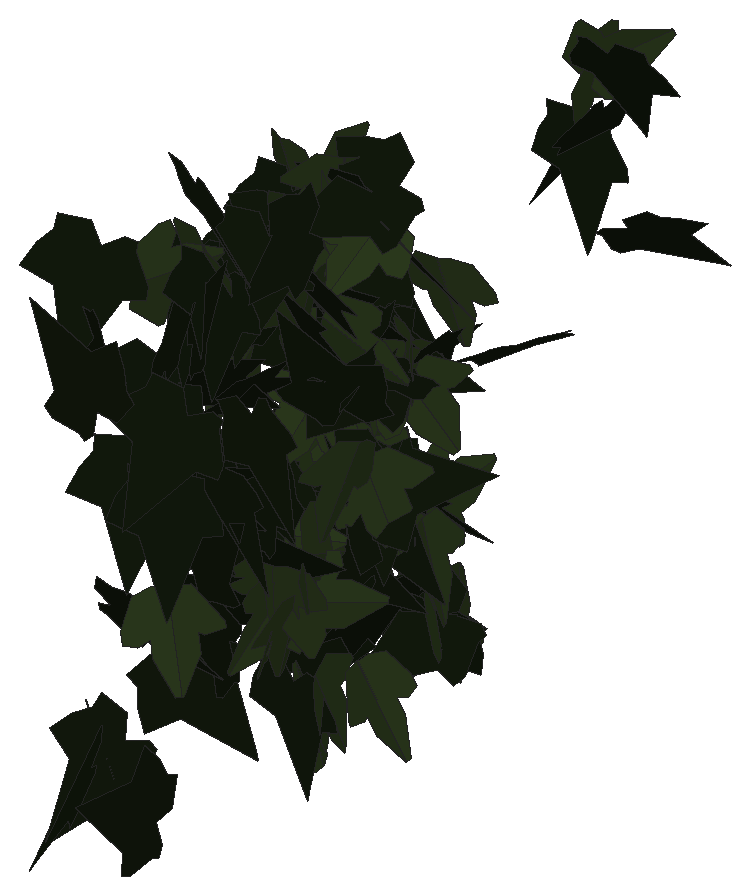
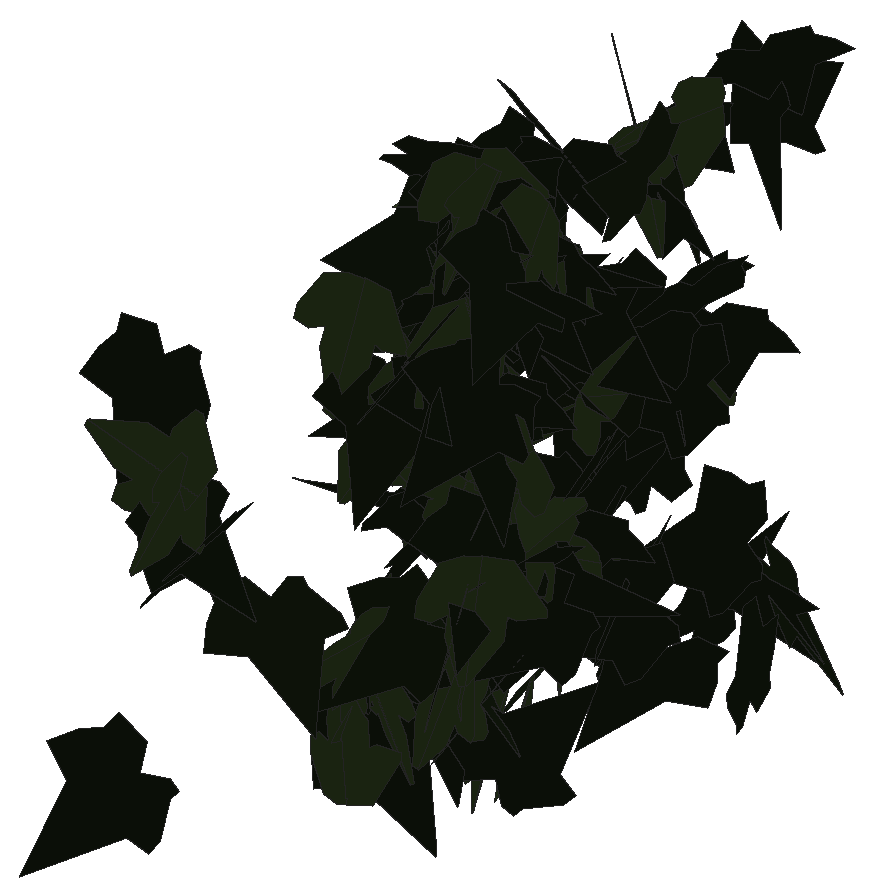
# SketchUp Ruby script. Lengths in inches.
U = 1.inch
M = Sketchup.active_model
def pt(a) = Geom::Point3d.new(a.map { |v| v * U })
def face(e, loops, mat)
  f = e.add_face(loops[0].map { |a| pt(a) })
  loops[1..].each { |l| e.add_face(l.map { |a| pt(a) }).erase! }
  f.material = f.back_material = mat if mat
  f
end
# faces: each face lists its corners as indices into pts; further lists are holes
def faces(e, pts, list, mat = nil) = list.each { |f| face(e, (f[0].is_a?(Array) ? f : [f]).map { |l| l.map { |i| pts[i] } }, mat) }
# xy, xz, yz: faces in a plane at the given z, y or x. An outline is a flat list of corners, or four numbers for a rectangle; further outlines are holes
def ring(l) = l.size == 4 ? [[l[0], l[1]], [l[2], l[1]], [l[2], l[3]], [l[0], l[3]]] : l.each_slice(2).to_a
def flat(e, list, mat, &to3) = list.each { |f| face(e, (f[0].is_a?(Array) ? f : [f]).map { |l| ring(l).map { |u, v| to3.(u, v) } }, mat) }
def xy(e, z, list, mat = nil) = flat(e, list, mat) { |x, y| [x, y, z] }
def xz(e, y, list, mat = nil) = flat(e, list, mat) { |x, z| [x, y, z] }
def yz(e, x, list, mat = nil) = flat(e, list, mat) { |y, z| [x, y, z] }
def lines(e, pts, list) = list.each { |a, b| e.add_line(pt(pts[a]), pt(pts[b])) }
# prism: a flat outline (further loops are holes) pulled along v
def prism(e, loops, v, mat = nil)
  f = face(e, loops, mat); d = Geom::Vector3d.new(v.map { |x| x * U })
  f.pushpull(f.normal.samedirection?(d) ? d.length : -d.length)
end
def box(e, o, s, mat = nil) = prism(e, [[o, [o[0] + s[0], o[1], o[2]], [o[0] + s[0], o[1] + s[1], o[2]], [o[0], o[1] + s[1], o[2]]]], [0, 0, s[2]], mat)
def at(x, y, z, deg = 0) = Geom::Transformation.translation(pt([x, y, z])) * Geom::Transformation.rotation(ORIGIN, Z_AXIS, deg.degrees)
def axes(o, x, y, z) = Geom::Transformation.new([*x, 0, *y, 0, *z, 0, *pt(o).to_a, 1])
def part(name) = M.definitions.add(name)
# library, detail: a bought-in or finely detailed component or shape, given as its bounding box
def library(name, o, s) = part(name).tap { |d| box(d.entities, o, s) }
def detail(e, o, s) = box(e.add_group.entities, o, s)
def put(e, d, t, mat = nil) = e.add_instance(d, t).tap { |i| i.material = mat if mat }
def group(e, t, mat = nil) = e.add_group.tap { |g| g.transformation = t; g.material = mat if mat }.entities
root = M.entities
M.materials.add("efeu1").color = [18, 25, 13]
M.materials.add("efeu2").color = [43, 57, 29]
c1 = part("ivyleaf_9")
p = [[1.54,2.16,1.25],[1.36,2.04,1.19],[-0.21,0.99,0.68],[-0.71,1.11,0.82],[-0.85,0.86,0.67],[-0.8,0.17,0.21],
  [-0.9,-0.01,0.1],[-0.67,-0.16,-0.02],[-0.08,-0.08,-0.05],[-0.03,-0.6,-0.4],[0.65,-0.88,-0.66],[0.83,-0.6,-0.49],
  [1.29,-0.42,-0.43],[1.8125,-0.07,-0.26],[1.21,0.44,0.15]]
faces(c1.entities,p,[[0,1,2,3,4,5,6,7,8,9,10,11,12,13,14]],"efeu1")
c2 = part("ivyleaf_10")
p = [[0,0.5,-0.03],[-0.0625,2.02,-0.43],[-0.19,2.01,-0.46],[-0.54,1.05,-0.29],[-0.52,0.625,-0.18],[-0.83,0.76,-0.28],
  [-1.16,0.64,-0.33],[-1.15,0.33,-0.24],[-0.77,-0.39,0.02],[-0.3,-0.51,0.16],[0.04,-0.48,0.23],[-0.02,2.01,-0.4375],
  [-0.06,2.01,-0.43],[0.04,-0.49,0.23],[0.67,-0.49,0.14],[1.38,0.36,-0.2],[1.375,0.51,-0.24],[0.81,0.65,-0.19],
  [0.62,0.59,-0.15],[0.6,1.09,-0.28],[0.5,1.23,-0.31]]
faces(c2.entities,p,[[0,1,2,3,4,5,6,7,8,9,10],[11,12,0,13,14,15,16,17,18,19,20]],"efeu2")
put(root,c1,axes([51.26,220.86,248.3],[0.28668,-0.3638,0.18833],[0.11725,-0.14738,-0.46318],[0.39252,0.30973,0.00081]))
put(root,c2,axes([51.57,222.2,244.75],[-0.11598,0.036,-0.48503],[-0.02936,-0.49824,-0.02996],[-0.48548,0.02153,0.11769]))
put(root,c1,axes([51.99,221.61,243.91],[-0.31629,0.04961,0.38406],[-0.38199,0.04146,-0.31994],[-0.06359,-0.4958,0.01167]))
put(root,c1,axes([51.36,223.23,243.51],[0.19328,-0.46108,0.00663],[0.00595,-0.0047,-0.49994],[0.46109,0.19334,0.00367]))
put(root,c2,axes([51.57,222.15,248.25],[-0.43953,0.21947,-0.09299],[0.07231,-0.0631,-0.4907],[-0.22712,-0.44481,0.02373]))
put(root,c2,axes([51.52,221.34,245.96],[-0.0779,-0.19546,0.45357],[0.19442,-0.43424,-0.15374],[0.45402,0.15241,0.14365]))
put(root,c1,axes([51.76,221.43,246.8],[-0.06436,0.17689,-0.46322],[0.04543,-0.46303,-0.18313],[-0.49375,-0.06566,0.04353]))
put(root,c1,axes([51.73,222.36,247.43],[-0.42644,-0.26019,-0.02116],[0.01619,0.01409,-0.49954],[0.26054,-0.42674,-0.00359]))
put(root,c1,axes([51.6,218.64,248.58],[-0.25307,-0.42792,-0.05328],[0.03038,0.04393,-0.49714],[0.43015,-0.25486,0.00377]))
put(root,c1,axes([51.46,219.9,246.58],[0.0908,-0.44479,-0.20957],[0.01331,0.21525,-0.4511],[0.49151,0.07635,0.05093]))
put(root,c2,axes([51.7,222.9,244.55],[-0.37664,-0.32541,-0.04743],[0.03783,0.02876,-0.49774],[0.32666,-0.37853,0.00296]))
put(root,c1,axes([51.77,222.17,247.75],[0.14094,0.44731,0.17335],[-0.02008,0.18602,-0.46368],[-0.4793,0.12374,0.0704]))
put(root,c1,axes([51.48,218.97,241.69],[-0.0454,-0.08304,0.49096],[0.13869,-0.4756,-0.06761],[0.47823,0.13005,0.06621]))
put(root,c1,axes([51.89,221.84,247.4375],[-0.40379,-0.19244,0.22343],[-0.14678,-0.19742,-0.43529],[0.25575,-0.41712,0.10294]))
put(root,c1,axes([51.32,219.3125,243.56],[0.42437,-0.11959,0.23581],[0.22597,-0.0675,-0.44089],[0.13728,0.48077,-0.00324]))
put(root,c1,axes([51.73,221.92,247.89],[-0.42595,-0.14972,-0.21483],[0.20764,0.05681,-0.45129],[0.15954,-0.47366,0.01378]))
put(root,c2,axes([52.01,220.06,247.96],[-0.39785,0.09308,0.28819],[-0.28916,0.02467,-0.40716],[-0.09001,-0.49064,0.0342]))
put(root,c1,axes([51.56,221.83,243.89],[0.41357,0.21089,0.1857],[0.15818,0.09838,-0.464],[-0.23224,0.44255,0.01466]))
put(root,c1,axes([51.67,220.26,247.77],[-0.33369,-0.1402,-0.34496],[0.34602,0.05436,-0.35681],[0.13755,-0.47685,0.06075]))
put(root,c1,axes([52.04,222.14,242],[0.16265,-0.00759,0.47275],[-0.46684,0.07659,0.16185],[-0.07488,-0.49404,0.01783]))
put(root,c1,axes([51.74,222.03,247.49],[-0.15012,0.09118,-0.46814],[0.34568,-0.31732,-0.17266],[-0.32859,-0.37549,0.03223]))
put(root,c1,axes([51.67,222.49,244.45],[-0.07447,-0.49405,0.01914],[0.05289,-0.0272,-0.49645],[0.49159,-0.07192,0.05632]))
put(root,c1,axes([51.63,220.11,242.6],[-0.01615,-0.25594,-0.42922],[0.07399,0.42349,-0.25531],[0.49423,-0.07177,0.0242]))
put(root,c1,axes([51.91,222.375,244.79],[0.15371,0.47271,0.05406],[-0.00337,0.05789,-0.49663],[-0.47577,0.15231,0.02098]))
put(root,c2,axes([51.51,222.42,245.81],[0.28931,-0.03294,0.40647],[0.40683,0.05764,-0.28489],[-0.02809,0.49557,0.06015]))
put(root,c1,axes([51.74,221.39,244.57],[-0.28529,-0.31507,-0.26332],[0.21986,0.1536,-0.42198],[0.3468,-0.35656,0.0509]))
put(root,c1,axes([51.75,220.09,246.3],[0.3452,0.3229,0.16302],[0.10935,0.12164,-0.47249],[-0.34479,0.36186,0.01336]))
put(root,c1,axes([51.5625,220.45,243.26],[0.40562,0.07389,0.28286],[0.27079,0.0874,-0.41114],[-0.1102,0.48672,0.03088]))
put(root,c1,axes([52.06,222.32,246.23],[-0.06487,0.49409,-0.04086],[0.01115,-0.03974,-0.49829],[-0.49565,-0.06556,-0.00586]))
put(root,c1,axes([51.73,228.15,244.72],[0.42356,0.23625,0.1216],[0.07732,0.10933,-0.48173],[-0.25421,0.42689,0.05608]))
put(root,c1,axes([52.05,217.88,242.33],[-0.38188,0.24669,-0.20811],[0.178,-0.10796,-0.4546],[-0.26923,-0.42129,-0.00536]))
put(root,c1,axes([51.95,220.89,244.33],[-0.10654,-0.15839,0.46213],[-0.20153,-0.41662,-0.18925],[0.44501,-0.22659,0.02493]))
put(root,c1,axes([51.78,220.84,245.13],[0.29553,-0.29838,-0.27135],[-0.16163,0.22059,-0.41859],[0.36951,0.33513,0.03393]))
put(root,c1,axes([52.15,218.03,247.79],[0.18574,0.03141,-0.46316],[-0.46216,-0.0344,-0.18768],[-0.04365,0.49783,0.01626]))
put(root,c1,axes([52.09,218.4375,242.45],[-0.47247,-0.16016,-0.03354],[0.03292,0.00734,-0.49886],[0.16029,-0.4736,0.00361]))
put(root,c2,axes([51.95,227.12,247.35],[-0.01205,-0.26423,-0.42431],[0.07235,0.41904,-0.26301],[0.49459,-0.06773,0.02813]))
put(root,c1,axes([52.04,222.67,244.3],[0.23102,-0.05226,-0.44034],[-0.39507,0.20122,-0.23115],[0.20137,0.45473,0.05168]))
put(root,c1,axes([51.89,219.03,245.73],[-0.31854,-0.31751,-0.21845],[0.16814,0.14052,-0.44942],[0.34679,-0.35978,0.01725]))
put(root,c1,axes([51.86,222.4375,246.45],[0.34188,0.34864,0.10756],[0.0691,0.08286,-0.48822],[-0.35825,0.34869,0.00847]))
put(root,c1,axes([51.91,220.52,245.91],[0.25705,0.31685,0.28902],[0.09313,0.28768,-0.3982],[-0.41863,0.25855,0.08888]))
put(root,c2,axes([51.83,219.25,248.07],[0.02127,-0.04023,-0.49792],[0.24173,0.43697,-0.02498],[0.43717,-0.23966,0.03804]))
put(root,c1,axes([52.11,219.22,247.04],[0.10233,0.07979,0.48287],[-0.06366,0.49129,-0.06769],[-0.48526,-0.04763,0.11071]))
put(root,c1,axes([51.96,220.5625,242.76],[-0.09802,0.00982,0.4902],[-0.12214,-0.48463,-0.01472],[0.47484,-0.12263,0.09741]))
put(root,c2,axes([52.0625,222.24,244.76],[-0.24033,-0.43536,0.05199],[0.01082,-0.06515,-0.49562],[0.43832,-0.2371,0.04074]))
put(root,c1,axes([51.76,219.38,245.18],[0.2831,0.11945,0.39445],[0.3145,0.24666,-0.30041],[-0.26636,0.4182,0.06452]))
put(root,c2,axes([51.96,221.76,247.84],[-0.47137,0.07466,-0.14912],[0.14341,-0.04673,-0.47671],[-0.08512,-0.49218,0.02264]))
put(root,c2,axes([51.97,221.51,247.5],[-0.46904,-0.04817,-0.16638],[0.17246,-0.08512,-0.46153],[0.01614,-0.49034,0.09646]))
put(root,c1,axes([51.99,222.3,246.36],[-0.32942,-0.28337,-0.24736],[0.19344,0.15436,-0.43446],[0.32259,-0.38194,0.00793]))
put(root,c1,axes([52.375,217.59,247.29],[0.0705,0.01386,0.49481],[-0.38445,0.31636,0.04592],[-0.31181,-0.38694,0.05526]))
put(root,c1,axes([52.25,226.92,246.97],[-0.21855,0.32414,-0.31172],[0.09747,-0.3042,-0.38466],[-0.43902,-0.2289,0.06978]))
put(root,c1,axes([51.84,221.69,247.38],[0.41578,-0.27673,-0.02335],[-0.02395,0.00614,-0.49939],[0.27668,0.41639,-0.00815]))
put(root,c2,axes([51.91,222.75,243.16],[0.00176,0.00965,0.4999],[0.31323,-0.38967,0.00642],[0.38972,0.31315,-0.00741]))
put(root,c2,axes([52.13,222.82,243.3],[-0.46407,0.17339,-0.06761],[0.06695,-0.01394,-0.4953],[-0.17365,-0.46877,-0.01028]))
put(root,c1,axes([51.97,226.96,246.55],[0.04959,-0.48818,0.09603],[0.03004,-0.09339,-0.49028],[0.49663,0.05439,0.02007]))
put(root,c1,axes([52.55,221.65,246.53],[-0.42631,0.13349,0.2246],[-0.20918,0.08314,-0.44646],[-0.15654,-0.47463,-0.01504]))
put(root,c2,axes([52.23,222.15,248.34],[-0.10709,0.38107,0.30548],[-0.1097,0.28598,-0.3952],[-0.47592,-0.15167,0.02236]))
put(root,c2,axes([52.21,222.38,247.12],[0.2655,0.40604,-0.12101],[-0.11442,-0.06879,-0.48185],[-0.40794,0.28355,0.05639]))
put(root,c2,axes([52.23,222.05,247.87],[0.27671,0.37306,-0.18507],[-0.11622,-0.1442,-0.46444],[-0.3999,0.30005,0.00691]))
put(root,c2,axes([52.19,221.78,245.47],[-0.31276,-0.18893,0.34131],[0.16621,-0.46029,-0.10249],[0.35293,0.04934,0.35072]))
put(root,c2,axes([51.91,221.17,243.97],[0.04759,-0.14933,-0.4748],[0.49585,0.05567,0.03219],[0.04325,-0.47392,0.15339]))
put(root,c2,axes([52.0625,227.1,247.41],[-0.21353,-0.21142,0.39963],[0.29474,0.27003,0.30034],[-0.34283,0.36385,0.00931]))
put(root,c1,axes([52.59,224.96,244.93],[-0.00337,0.48882,-0.10508],[-0.20225,-0.09743,-0.44677],[-0.45726,0.0395,0.19838]))
put(root,c2,axes([52.43,222.03,248.41],[-0.3809,-0.31944,0.05355],[-0.03692,-0.03931,-0.49708],[0.32179,-0.38264,0.00636]))
put(root,c1,axes([52.08,222.33,245],[0.11628,-0.37991,0.30356],[0.09467,-0.28846,-0.39728],[0.47699,0.14987,0.00485]))
put(root,c1,axes([52.29,221.95,248.28],[0.44401,0.17074,-0.15397],[-0.14537,-0.05093,-0.47568],[-0.17812,0.46718,0.00441]))
put(root,c1,axes([52.11,219.74,244.18],[-0.12351,0.01114,0.48438],[0.33492,-0.35924,0.09366],[0.35011,0.34759,0.08128]))
put(root,c2,axes([52.48,220.72,243.25],[0.19398,-0.38193,-0.25787],[-0.08536,0.24517,-0.42732],[0.45287,0.20981,0.02991]))
put(root,c1,axes([52.4,220.68,248.08],[-0.36743,-0.29294,-0.17083],[0.14231,0.09544,-0.46972],[0.30781,-0.3938,0.01324]))
put(root,c1,axes([52.76,220.35,244.73],[-0.04003,0.03925,0.49685],[-0.32741,0.37373,-0.0559],[-0.37576,-0.32983,-0.00421]))
put(root,c2,axes([52.5,221.27,247.24],[0.01912,-0.49947,0.01288],[-0.00464,-0.01306,-0.49981],[0.49961,0.019,-0.00513]))
put(root,c1,axes([52.31,219.49,247.3],[-0.10787,0.30262,0.38313],[0.08094,-0.37585,0.31966],[0.48147,0.13098,0.03209]))
put(root,c1,axes([52.29,219.93,247.83],[0.01876,-0.48647,0.11398],[0.01419,-0.11349,-0.48674],[0.49945,0.0215,0.00955]))
put(root,c1,axes([52.78,222.08,243.34],[-0.35042,0.35405,0.04309],[-0.03887,0.02213,-0.498],[-0.35454,-0.35236,0.01202]))
put(root,c2,axes([52.53,220.73,243.45],[0.0766,0.29903,-0.39334],[-0.12312,-0.37393,-0.30825],[-0.47851,0.14408,0.01634]))
put(root,c2,axes([52.64,220.54,243.84],[-0.46703,-0.17385,0.04069],[-0.03597,-0.01999,-0.4983],[0.17489,-0.46838,0.00617]))
put(root,c2,axes([52.35,222.29,245.03],[0.44714,0.1249,0.18566],[0.17503,0.06322,-0.46408],[-0.1394,0.48,0.01281]))
put(root,c1,axes([52.52,222.36,247.24],[-0.21886,-0.44921,0.01771],[0.01017,-0.02464,-0.49929],[0.44944,-0.21818,0.01992]))
put(root,c1,axes([52.34,220.93,247.23],[0.49735,-0.04345,-0.02755],[-0.02725,0.00463,-0.49924],[0.04364,0.49809,0.00224]))
put(root,c1,axes([52.35,222.96,243.875],[0.49185,0.06989,0.05654],[0.0422,0.09822,-0.48844],[-0.07938,0.48525,0.09072]))
put(root,c1,axes([52.43,222.4,247.02],[0.30693,-0.2732,-0.28488],[-0.12078,0.27856,-0.39726],[0.37577,0.31268,0.105]))
put(root,c2,axes([52.71,221.14,241.46],[-0.2052,0.45084,-0.06805],[-0.03799,0.05746,0.49523],[0.45437,0.20842,0.01067]))
put(root,c1,axes([52.28,221.73,243.62],[0.02211,0.0454,-0.49744],[0.30806,0.39072,0.04936],[0.39321,-0.30866,-0.01069]))
put(root,c1,axes([52.68,218.27,241.73],[-0.04028,-0.02414,0.49779],[-0.2589,-0.42573,-0.04159],[0.42585,-0.2611,0.02179]))
put(root,c2,axes([52.76,223.12,243.18],[0.38683,-0.22506,-0.22295],[-0.17791,0.13682,-0.4468],[0.26212,0.425,0.02577]))
put(root,c1,axes([52.41,219.875,245.39],[0.25741,-0.42864,0.00309],[0.00043,-0.00334,-0.49999],[0.42865,0.25741,-0.00135]))
put(root,c1,axes([52.42,221.47,246.99],[0.45884,0.14378,0.13709],[0.12035,0.07331,-0.47973],[-0.15805,0.47324,0.03267]))
put(root,c2,axes([52.71,220.77,243.42],[0.05781,-0.49662,0.00469],[0.00271,-0.00441,-0.49997],[0.49664,0.05783,0.00218]))
put(root,c1,axes([52.55,218.77,245.7],[-0.06614,-0.49369,-0.04356],[0.00564,0.04319,-0.4981],[0.49557,-0.06638,-0.00015]))
put(root,c2,axes([52.74,221.31,242.1],[-0.16167,0.42183,0.2143],[-0.12658,0.17965,-0.44911],[-0.45589,-0.19947,0.04871]))
put(root,c1,axes([52.29,220.64,244.05],[0.14779,-0.18467,0.44051],[0.40939,-0.18858,-0.21641],[0.24608,0.42465,0.09546]))
put(root,c1,axes([52.87,222.07,242.98],[-0.02076,0.48289,-0.128],[0.01699,-0.12735,-0.48321],[-0.49928,-0.02441,-0.01112]))
put(root,c1,axes([52.99,220.63,248.4],[-0.47735,0.14058,-0.0487],[0.04526,-0.01867,-0.4976],[-0.14173,-0.47947,0.0051]))
put(root,c1,axes([53.01,222.11,246.08],[-0.48579,-0.092,0.07447],[-0.07533,-0.00232,-0.49429],[0.0913,-0.49146,-0.0116]))
put(root,c2,axes([52.76,223.32,243.72],[0.14182,0.01797,-0.47913],[0.11275,0.48439,0.05153],[0.46602,-0.12266,0.13334]))
put(root,c1,axes([52.52,222.25,246.03],[0.16938,-0.03691,-0.46899],[0.14957,0.47682,0.01649],[0.44603,-0.14588,0.17257]))
put(root,c1,axes([52.6,220.93,242.29],[0.09851,-0.47136,0.1346],[0.05386,-0.12605,-0.48084],[0.48723,0.10924,0.02594]))
put(root,c1,axes([53.11,222.09,248.42],[-0.45182,-0.07812,0.1994],[-0.17779,-0.12269,-0.45093],[0.11938,-0.47838,0.08308]))
put(root,c1,axes([52.61,220.17,246.07],[0.22118,-0.44713,-0.03396],[-0.01142,0.03224,-0.49883],[0.44827,0.22143,0.00405]))
put(root,c2,axes([52.87,220.84,244.14],[0.1199,-0.19959,-0.44248],[0.0082,0.45655,-0.20371],[0.48534,0.04159,0.11276]))
put(root,c1,axes([52.83,226.36,248.14],[0.41987,0.18503,-0.19867],[-0.17541,-0.09437,-0.45861],[-0.20721,0.45482,-0.01433]))
put(root,c1,axes([53.1,222.79,242.5],[0.15279,0.23609,-0.41342],[-0.239,-0.33747,-0.28105],[-0.41174,0.2835,0.00973]))
put(root,c2,axes([52.96,221.95,247.8125],[-0.49788,-0.03148,0.03351],[0.02699,-0.49513,-0.06418],[0.03722,-0.06209,0.49473]))
put(root,c1,axes([52.84,220.69,247.86],[0.47118,0.05305,-0.15867],[-0.16197,0.02591,-0.47233],[-0.04189,0.4965,0.0416]))
put(root,c2,axes([53.02,222.34,246.07],[-0.16766,-0.44774,0.14634],[-0.00556,-0.15344,-0.47584],[0.47102,-0.16119,0.04647]))
put(root,c1,axes([53.08,222.5,245.96],[0.10217,0.47271,0.12689],[-0.00057,0.12974,-0.48287],[-0.48945,0.09853,0.02705]))
put(root,c2,axes([52.93,223.36,242.1875],[-0.47662,0.03841,0.14614],[0.14569,-0.01145,0.47817],[0.04008,0.49839,-0.00027]))
put(root,c2,axes([52.81,220.88,243.49],[0.00747,-0.15363,-0.47576],[0.32042,0.36671,-0.11338],[0.38376,-0.30319,0.10393]))
put(root,c1,axes([52.88,222.1875,244.8],[-0.11824,-0.47268,-0.11223],[0.05889,0.10071,-0.4862],[0.48224,-0.12819,0.03185]))
put(root,c2,axes([52.87,218.29,244.54],[0.44439,0.18474,0.13561],[0.12959,0.04144,-0.48113],[-0.18901,0.46277,-0.01106]))
put(root,c1,axes([53.1,218.3,247.07],[-0.27791,-0.41013,0.06749],[-0.04133,-0.05352,-0.49541],[0.41359,-0.28094,-0.00416]))
put(root,c1,axes([53.36,222.83,242.6],[-0.46791,-0.12654,0.12266],[-0.11194,-0.05539,-0.48415],[0.13612,-0.48054,0.02351]))
put(root,c1,axes([53.41,221.29,246.76],[-0.37151,0.3346,-0.00504],[0.00383,-0.00329,-0.49997],[-0.33461,-0.37153,-0.00012]))
put(root,c1,axes([53.3,220.89,246.19],[0.28975,-0.05918,0.40316],[-0.39268,0.09157,0.29566],[-0.10883,-0.48797,0.00659]))
put(root,c1,axes([52.98,221.9,244.35],[0.25363,-0.33578,-0.27005],[-0.09163,0.26416,-0.41452],[0.42104,0.25975,0.07247]))
put(root,c2,axes([53.16,222.23,246.28],[0.3803,-0.316,-0.0743],[0.03021,0.1484,-0.47651],[0.32321,0.35794,0.13197]))
put(root,c2,axes([53.1875,222.77,242.71],[-0.18885,0.45321,0.09453],[-0.02617,0.09148,-0.49086],[-0.46223,-0.19034,-0.01083]))
put(root,c1,axes([52.83,222.34,247.61],[0.37154,-0.26215,0.20793],[0.18771,-0.09393,-0.45381],[0.27699,0.41528,0.02862]))
put(root,c2,axes([53.04,222.45,245.67],[0.26877,0.31206,0.28352],[0.1275,0.26033,-0.4074],[-0.40188,0.29129,0.06037]))
put(root,c2,axes([53.11,221.66,244.83],[0.24673,0.39913,0.17269],[0.04058,0.17655,-0.46603],[-0.43298,0.24399,0.05473]))
put(root,c2,axes([53.26,221.1,245.37],[-0.03499,-0.46761,0.17355],[0.03103,-0.17568,-0.46709],[0.49781,-0.02192,0.04132]))
put(root,c2,axes([53.19,222.64,243.63],[-0.1163,0.48611,-0.01295],[0.00341,-0.0125,-0.49983],[-0.48627,-0.11635,-0.00041]))
put(root,c1,axes([52.88,221.99,244.52],[0.43278,-0.14843,-0.20166],[0.16183,0.47309,-0.0009],[0.19108,-0.06449,0.45753]))
put(root,c2,axes([53.28,222.81,247.05],[-0.49664,-0.04057,-0.0413],[0.04125,0.00236,-0.49829],[0.04063,-0.49835,0.001]))
put(root,c1,axes([53.35,221.96,246.17],[-0.4558,-0.14216,0.14845],[0.08629,-0.46011,-0.17565],[0.18655,-0.1345,0.44397]))
put(root,c2,axes([53.05,221.76,242.15],[-0.34792,-0.00447,-0.35907],[0.31858,-0.23455,-0.30577],[-0.1657,-0.44155,0.16606]))
put(root,c2,axes([52.95,221.37,246.85],[-0.19548,0.05675,-0.45669],[0.44232,-0.11382,-0.20347],[-0.12706,-0.48355,-0.0057]))
